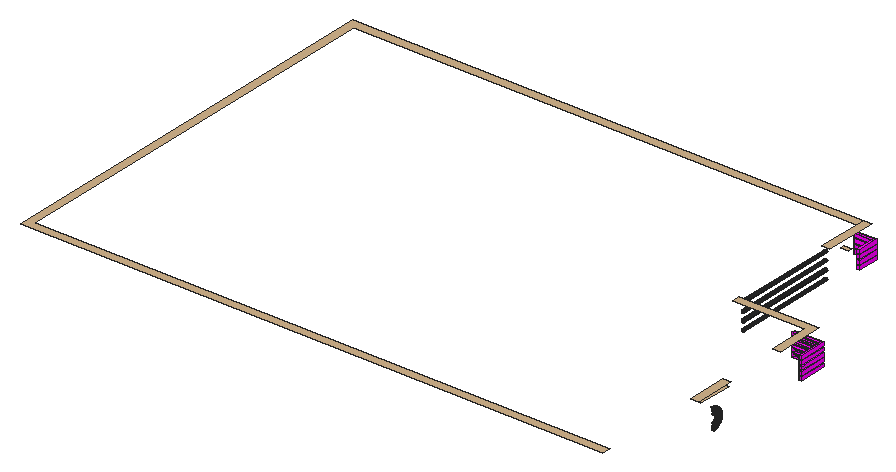
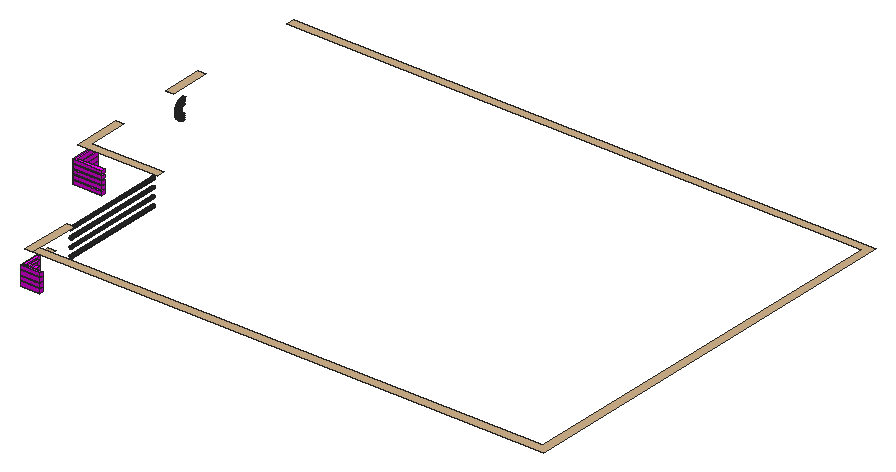
# SketchUp Ruby script. Lengths in inches.
U = 1.inch
M = Sketchup.active_model
def pt(a) = Geom::Point3d.new(a.map { |v| v * U })
def face(e, loops, mat)
  f = e.add_face(loops[0].map { |a| pt(a) })
  loops[1..].each { |l| e.add_face(l.map { |a| pt(a) }).erase! }
  f.material = f.back_material = mat if mat
  f
end
# faces: each face lists its corners as indices into pts; further lists are holes
def faces(e, pts, list, mat = nil) = list.each { |f| face(e, (f[0].is_a?(Array) ? f : [f]).map { |l| l.map { |i| pts[i] } }, mat) }
# xy, xz, yz: faces in a plane at the given z, y or x. An outline is a flat list of corners, or four numbers for a rectangle; further outlines are holes
def ring(l) = l.size == 4 ? [[l[0], l[1]], [l[2], l[1]], [l[2], l[3]], [l[0], l[3]]] : l.each_slice(2).to_a
def flat(e, list, mat, &to3) = list.each { |f| face(e, (f[0].is_a?(Array) ? f : [f]).map { |l| ring(l).map { |u, v| to3.(u, v) } }, mat) }
def xy(e, z, list, mat = nil) = flat(e, list, mat) { |x, y| [x, y, z] }
def xz(e, y, list, mat = nil) = flat(e, list, mat) { |x, z| [x, y, z] }
def yz(e, x, list, mat = nil) = flat(e, list, mat) { |y, z| [x, y, z] }
def lines(e, pts, list) = list.each { |a, b| e.add_line(pt(pts[a]), pt(pts[b])) }
# prism: a flat outline (further loops are holes) pulled along v
def prism(e, loops, v, mat = nil)
  f = face(e, loops, mat); d = Geom::Vector3d.new(v.map { |x| x * U })
  f.pushpull(f.normal.samedirection?(d) ? d.length : -d.length)
end
def box(e, o, s, mat = nil) = prism(e, [[o, [o[0] + s[0], o[1], o[2]], [o[0] + s[0], o[1] + s[1], o[2]], [o[0], o[1] + s[1], o[2]]]], [0, 0, s[2]], mat)
def at(x, y, z, deg = 0) = Geom::Transformation.translation(pt([x, y, z])) * Geom::Transformation.rotation(ORIGIN, Z_AXIS, deg.degrees)
def axes(o, x, y, z) = Geom::Transformation.new([*x, 0, *y, 0, *z, 0, *pt(o).to_a, 1])
def part(name) = M.definitions.add(name)
# library, detail: a bought-in or finely detailed component or shape, given as its bounding box
def library(name, o, s) = part(name).tap { |d| box(d.entities, o, s) }
def detail(e, o, s) = box(e.add_group.entities, o, s)
def put(e, d, t, mat = nil) = e.add_instance(d, t).tap { |i| i.material = mat if mat }
def group(e, t, mat = nil) = e.add_group.tap { |g| g.transformation = t; g.material = mat if mat }.entities
root = M.entities
M.materials.add("[0035_Tan]").color = [210, 180, 140]
M.materials.add("[0127_Magenta]").color = [255, 0, 255]
M.materials.add("[0136_Charcoal]").color = [35, 35, 35]
c1 = part("Component\#10")
xy(c1.entities,0,[[20,0,20,19,0,19,0,21,22,21,22,0]])
xy(c1.entities,2.5625,[[20,0,22,0,22,21,0,21,0,19,20,19]])
xz(c1.entities,0,[[20,0,22,2.5625]])
xz(c1.entities,21,[[0,0,22,2.5625]])
yz(c1.entities,0,[[19,0,21,2.5625]])
yz(c1.entities,20,[[0,0,19,2.5625]])
yz(c1.entities,22,[[0,0,21,2.5625]])
c2 = part("Group\#24")
prism(c2.entities,[[[2.25,1.125,0],[2.21,0.83,0],[2.1,0.5625,0],[1.92,0.33,0],[1.6875,0.15,0],[1.42,0.04,0],[1.125,0,0],[0.83,0.04,0],[0.5625,0.15,0],[0.33,0.33,0],[0.15,0.5625,0],[0.04,0.83,0],[0,1.125,0],[0.04,1.42,0],[0.15,1.6875,0],[0.33,1.92,0],[0.5625,2.1,0],[0.83,2.21,0],[1.125,2.25,0],[1.42,2.21,0],[1.6875,2.1,0],[1.92,1.92,0],[2.1,1.6875,0],[2.21,1.42,0]]],[0,0,77.9])
c3 = part("Component\#2")
xy(c3.entities,-13,[[13.51,0,15.51,2.94]],"[0127_Magenta]")
xy(c3.entities,2,[[0,0,15.51,2.94]],"[0127_Magenta]")
xz(c3.entities,0,[[13.51,-13,15.51,0],[0,0,15.51,2]],"[0127_Magenta]")
xz(c3.entities,2.94,[[13.51,-13,15.51,2],[0,0,13.51,2]],"[0127_Magenta]")
yz(c3.entities,0,[[0,0,2.94,2]],"[0127_Magenta]")
yz(c3.entities,13.51,[[0,-13,2.94,2]],"[0127_Magenta]")
yz(c3.entities,15.51,[[0,-13,2.94,2]],"[0127_Magenta]")
xy(root,161.91,[[442,98.56,443.75,98.95]],"[0035_Tan]")
xy(root,163.37,[[442,98.52,443.75,99]],"[0127_Magenta]")
xy(root,165.21,[[384,292.3,390,295.12]],"[0035_Tan]")
xy(root,172,[[442,86.55,444,112.55]],"[0035_Tan]")
xy(root,174,[[0,2,438,2,438,8,6,8,6,308,384,308,384,314,0,314],[438,84.55,444,114.55],[438,161.1,444,161.1,444,197.1,384,197.1,384,191.1,438,191.1],[384,275,390,314]],"[0035_Tan]")
xz(root,101.97,[[442,155.57,443.5,155.77]],"[0035_Tan]")
xz(root,103.75,[[442,155.51,443.5,155.82]],"[0127_Magenta]")
xz(root,104.99,[[442,155.47,443.75,155.86]],"[0035_Tan]")
xz(root,106.44,[[442,155.42,443.75,155.91]],"[0127_Magenta]")
p = [[442,98.98,147.98],[442,99.47,148.01],[443.75,99.47,148.01],[443.75,98.98,147.98],[442,99.95,148.07],[443.75,99.95,148.07],
  [442,100.42,148.16],[443.75,100.42,148.16],[442,100.89,148.28],[443.75,100.89,148.28],[442,101.35,148.43],[443.75,101.35,148.43],
  [442,101.8,148.61],[443.75,101.8,148.61],[442,102.24,148.8125],[443.75,102.24,148.8125],[442,102.66,149.04],[443.75,102.66,149.04],
  [442,103.07,149.3],[443.75,103.07,149.3],[442,103.46,149.59],[443.75,103.46,149.59],[442,99.33,149.46],[442,98.9375,149.43],
  [443.75,98.9375,149.43],[443.75,99.33,149.46],[442,99.72,149.51],[443.75,99.72,149.51],[442,100.1,149.58],[443.75,100.1,149.58],
  [442,100.48,149.68],[443.75,100.48,149.68],[442,103.83,149.89],[443.75,103.83,149.89],[442,100.86,149.8],[443.75,100.86,149.8],
  [442,101.22,149.94],[443.75,101.22,149.94],[442,101.58,150.11],[443.75,101.58,150.11],[442,104.1875,150.22],[443.75,104.1875,150.22],
  [442,101.92,150.3],[443.75,101.92,150.3],[442,104.52,150.58],[443.75,104.52,150.58],[442,102.25,150.51],[443.75,102.25,150.51],
  [442,102.57,150.74],[443.75,102.57,150.74],[442,104.83,150.95],[443.75,104.83,150.95],[442,98.9,150.68],[442,99.21,150.69],
  [443.5,99.21,150.69],[443.5,98.9,150.68],[442,99.53,150.73],[443.5,99.53,150.73],[442,99.84,150.79],[443.5,99.84,150.79],
  [442,102.87,150.99],[443.75,102.87,150.99],[442,100.14,150.87],[443.5,100.14,150.87],[442,100.4375,150.97],[443.5,100.4375,150.97],
  [442,105.11,151.34],[443.75,105.11,151.34],[442,100.73,151.08],[443.5,100.73,151.08],[442,103.16,151.26],[443.75,103.16,151.26],
  [442,101.01,151.22],[443.5,101.01,151.22],[442,101.29,151.37],[443.5,101.29,151.37],[442,103.43,151.54],[443.75,103.43,151.54],
  [442,105.37,151.75],[443.75,105.37,151.75],[442,101.56,151.53],[443.5,101.56,151.53],[442,101.81,151.72],[443.5,101.81,151.72],
  [442,103.68,151.84],[443.75,103.68,151.84],[442,102.05,151.92],[443.5,102.05,151.92],[442,105.6,152.17],[443.75,105.6,152.17],
  [442,103.91,152.16],[443.75,103.91,152.16],[442,102.28,152.13],[443.5,102.28,152.13],[442,102.5,152.36],[443.5,102.5,152.36],
  [442,104.12,152.49],[443.75,104.12,152.49],[442,105.81,152.61],[443.75,105.81,152.61],[442,99.05,152.46],[442,98.85,152.45],
  [443.5,98.85,152.45],[443.5,99.05,152.46],[442,102.7,152.6],[443.5,102.7,152.6],[442,99.25,152.49],[443.5,99.25,152.49],
  [442,99.45,152.52],[443.5,99.45,152.52],[442,99.65,152.57],[443.5,99.65,152.57],[442,104.31,152.83],[443.75,104.31,152.83],
  [442,99.84,152.64],[443.5,99.84,152.64],[442,100.03,152.71],[443.5,100.03,152.71],[442,102.88,152.86],[443.5,102.88,152.86],
  [442,105.99,153.06],[443.75,105.99,153.06],[442,100.21,152.8],[443.5,100.21,152.8],[442,100.39,152.9],[443.5,100.39,152.9],
  [442,104.47,153.1875],[443.75,104.47,153.1875],[442,100.56,153],[443.5,100.56,153],[442,103.05,153.12],[443.5,103.05,153.12],
  [442,100.72,153.12],[443.5,100.72,153.12],[442,100.88,153.25],[443.5,100.88,153.25],[442,103.2,153.4],[443.5,103.2,153.4],
  [442,106.14,153.52],[443.75,106.14,153.52],[442,104.62,153.55],[443.75,104.62,153.55],[442,101.03,153.39],[443.5,101.03,153.39],
  [442,101.17,153.54],[443.5,101.17,153.54],[442,103.34,153.68],[443.5,103.34,153.68],[442,101.3,153.69],[443.5,101.3,153.69],
  [442,106.26,153.99],[443.75,106.26,153.99],[442,104.74,153.93],[443.75,104.74,153.93],[442,101.41,153.86],[443.5,101.41,153.86],
  [442,103.45,153.97],[443.5,103.45,153.97],[442,101.52,154.03],[443.5,101.52,154.03],[442,104.84,154.3],[443.75,104.84,154.3],
  [442,101.62,154.21],[443.5,101.62,154.21],[442,103.55,154.27],[443.5,103.55,154.27],[442,106.35,154.46],[443.75,106.35,154.46],
  [442,101.71,154.39],[443.5,101.71,154.39],[442,103.63,154.58],[443.5,103.63,154.58],[442,104.91,154.69],[443.75,104.91,154.69],
  [442,101.78,154.58],[443.5,101.78,154.58],[442,106.41,154.94],[443.75,106.41,154.94],[442,101.85,154.77],[443.5,101.85,154.77],
  [442,103.6875,154.89],[443.5,103.6875,154.89],[442,104.96,155.08],[443.75,104.96,155.08],[442,101.9,154.97],[443.5,101.9,154.97],
  [442,103.73,155.2],[443.5,103.73,155.2],[442,106.44,155.42],[443.75,106.44,155.42],[442,101.93,155.16],[443.5,101.93,155.16],
  [442,104.99,155.47],[443.75,104.99,155.47],[442,101.96,155.37],[443.5,101.96,155.37],[442,103.75,155.51],[443.5,103.75,155.51],
  [442,101.97,155.57],[443.5,101.97,155.57],[442,101.96,155.97],[442,101.97,155.77],[443.5,101.97,155.77],[443.5,101.96,155.97],
  [442,103.75,155.82],[442,103.73,156.14],[443.5,103.73,156.14],[443.5,103.75,155.82],[442,104.96,156.25],[442,104.99,155.86],
  [443.75,104.99,155.86],[443.75,104.96,156.25],[442,106.44,155.91],[442,106.41,156.39],[443.75,106.41,156.39],[443.75,106.44,155.91],
  [442,101.94,156.17],[443.5,101.94,156.17],[442,103.6875,156.45],[443.5,103.6875,156.45],[442,101.9,156.37],[443.5,101.9,156.37],
  [442,104.91,156.64],[443.75,104.91,156.64],[442,101.85,156.57],[443.5,101.85,156.57],[442,103.63,156.76],[443.5,103.63,156.76],
  [442,106.35,156.87],[443.75,106.35,156.87],[442,101.78,156.76],[443.5,101.78,156.76],[442,104.84,157.03],[443.75,104.84,157.03],
  [442,101.71,156.95],[443.5,101.71,156.95],[442,103.55,157.0625],[443.5,103.55,157.0625],[442,106.26,157.34],[443.75,106.26,157.34],
  [442,101.625,157.13],[443.5,101.625,157.13],[442,104.74,157.41],[443.75,104.74,157.41],[442,101.53,157.3125],[443.5,101.53,157.3125],
  [442,103.46,157.36],[443.5,103.46,157.36],[442,101.42,157.48],[443.5,101.42,157.48],[442,106.14,157.8125],[443.75,106.14,157.8125],
  [442,103.34,157.65],[443.5,103.34,157.65],[442,104.625,157.78],[443.75,104.625,157.78],[442,101.3,157.65],[443.5,101.3,157.65],
  [442,101.17,157.8],[443.5,101.17,157.8],[442,103.21,157.9375],[443.5,103.21,157.9375],[442,101.03,157.95],[443.5,101.03,157.95],
  [442,104.48,158.15],[443.75,104.48,158.15],[442,105.99,158.27],[443.75,105.99,158.27],[442,103.06,158.21],[443.5,103.06,158.21],
  [442,100.88,158.09],[443.5,100.88,158.09],[442,100.73,158.22],[443.5,100.73,158.22],[442,104.3125,158.5],[443.75,104.3125,158.5],
  [442,100.57,158.34],[443.5,100.57,158.34],[442,102.89,158.48],[443.5,102.89,158.48],[442,100.39,158.45],[443.5,100.39,158.45],
  [442,105.82,158.72],[443.75,105.82,158.72],[442,100.22,158.54],[443.5,100.22,158.54],[442,100.03,158.63],[443.5,100.03,158.63],
  [442,102.7,158.73],[443.5,102.7,158.73],[442,104.125,158.84],[443.75,104.125,158.84],[442,99.85,158.71],[443.5,99.85,158.71],
  [442,99.65,158.77],[443.5,99.65,158.77],[442,102.5,158.98],[443.5,102.5,158.98],[442,105.61,159.16],[443.75,105.61,159.16],
  [442,99.26,158.86],[442,99.46,158.82],[443.5,99.46,158.82],[443.5,99.26,158.86],[442,103.92,159.18],[443.75,103.92,159.18],
  [442,98.85,158.9],[442,99.06,158.88],[443.5,99.06,158.88],[443.5,98.85,158.9],[442,102.29,159.2],[443.5,102.29,159.2],
  [442,102.06,159.42],[443.5,102.06,159.42],[442,103.69,159.49],[443.75,103.69,159.49],[442,105.38,159.58],[443.75,105.38,159.58],
  [442,101.82,159.62],[443.5,101.82,159.62],[442,103.44,159.79],[443.75,103.44,159.79],[442,101.5625,159.81],[443.5,101.5625,159.81],
  [442,105.12,159.99],[443.75,105.12,159.99],[442,101.3,159.97],[443.5,101.3,159.97],[442,103.17,160.08],[443.75,103.17,160.08],
  [442,101.02,160.125],[443.5,101.02,160.125],[442,104.84,160.38],[443.75,104.84,160.38],[442,100.74,160.26],[443.5,100.74,160.26],
  [442,102.88,160.35],[443.75,102.88,160.35],[442,100.45,160.375],[443.5,100.45,160.375],[442,102.58,160.6],[443.75,102.58,160.6],
  [442,100.15,160.47],[443.5,100.15,160.47],[442,104.53,160.76],[443.75,104.53,160.76],[442,99.85,160.55],[443.5,99.85,160.55],
  [442,99.54,160.61],[442,99.23,160.65],[443.5,99.23,160.65],[443.5,99.54,160.61],[442,102.26,160.83],[443.75,102.26,160.83],
  [442,98.91,160.67],[443.5,98.91,160.67],[442,101.93,161.04],[443.75,101.93,161.04],[442,104.2,161.11],[443.75,104.2,161.11],
  [442,101.59,161.23],[443.75,101.59,161.23],[442,103.85,161.44],[443.75,103.85,161.44],[442,101.23,161.4],[443.75,101.23,161.4],
  [442,100.87,161.54],[443.75,100.87,161.54],[442,103.47,161.75],[443.75,103.47,161.75],[442,100.5,161.66],[443.75,100.5,161.66],
  [442,100.12,161.76],[443.75,100.12,161.76],[442,103.08,162.03],[443.75,103.08,162.03],[442,99.34,161.89],[442,99.73,161.84],
  [443.75,99.73,161.84],[443.75,99.34,161.89],[442,98.95,161.91],[443.75,98.95,161.91],[442,102.67,162.29],[443.75,102.67,162.29],
  [442,102.25,162.53],[443.75,102.25,162.53],[442,101.8125,162.73],[443.75,101.8125,162.73],[442,101.36,162.91],[443.75,101.36,162.91],
  [442,100.9,163.0625],[443.75,100.9,163.0625],[442,100.4375,163.18],[443.75,100.4375,163.18],[442,99.96,163.27],[443.75,99.96,163.27],
  [442,99.48,163.33],[442,99,163.37],[443.75,99,163.37],[443.75,99.48,163.33]]
faces(root,p,[[0,1,2,3],[1,4,5,2],[4,6,7,5],[6,8,9,7],[8,10,11,9],[10,12,13,11],[12,14,15,13],[14,16,17,15],
  [16,18,19,17],[18,20,21,19],[20,32,33,21],[32,40,41,33],[40,44,45,41],[44,50,51,45],[52,53,54,55],[53,56,57,54],
  [56,58,59,57],[58,62,63,59],[62,64,65,63],[50,66,67,51],[64,68,69,65],[68,72,73,69],[72,74,75,73],[66,78,79,67],
  [74,80,81,75],[80,82,83,81],[82,86,87,83],[78,88,89,79],[86,92,93,87],[92,94,95,93],[88,98,99,89],[94,104,105,95],
  [104,118,119,105],[98,120,121,99],[118,130,131,119],[130,136,137,131],[120,138,139,121],[136,146,147,137],[138,150,151,139],[146,156,157,147],
  [156,164,165,157],[150,166,167,151],[164,170,171,165],[166,176,177,167],[170,180,181,171],[180,186,187,181],[176,188,189,177],[186,196,197,187],
  [204,205,206,207],[212,213,214,215],[205,218,219,206],[218,226,227,219],[213,228,229,214],[226,236,237,227],[228,238,239,229],[236,246,247,237],
  [238,250,251,239],[246,252,253,247],[252,260,261,253],[250,266,267,251],[260,268,269,261],[268,278,279,269],[266,282,283,267],[278,288,289,279],
  [288,296,297,289],[282,298,299,283],[296,310,311,297],[310,312,313,311],[298,316,317,299],[312,318,319,313],[318,322,323,319],[316,324,325,317],
  [322,326,327,323],[326,330,331,327],[324,332,333,325],[330,334,335,331],[334,338,339,335],[338,342,343,339],[332,344,345,333],[342,346,347,343],
  [348,349,350,351],[346,348,351,347],[349,354,355,350],[344,358,359,345],[358,362,363,359],[362,368,369,363],[368,374,375,369],[374,382,383,375],
  [382,384,385,383],[384,386,387,385],[386,388,389,387],[388,390,391,389],[390,392,393,391],[392,394,395,393],[396,397,398,399],[394,396,399,395]],"[0127_Magenta]")
faces(root,p,[[22,23,24,25],[26,22,25,27],[28,26,27,29],[30,28,29,31],[34,30,31,35],[36,34,35,37],[38,36,37,39],[42,38,39,43],
  [46,42,43,47],[48,46,47,49],[60,48,49,61],[70,60,61,71],[76,70,71,77],[84,76,77,85],[90,84,85,91],[96,90,91,97],
  [100,101,102,103],[106,100,103,107],[108,106,107,109],[110,108,109,111],[112,96,97,113],[114,110,111,115],[116,114,115,117],[122,116,117,123],
  [124,122,123,125],[126,112,113,127],[128,124,125,129],[132,128,129,133],[134,132,133,135],[140,126,127,141],[142,134,135,143],[144,142,143,145],
  [148,144,145,149],[152,140,141,153],[154,148,149,155],[158,154,155,159],[160,152,153,161],[162,158,159,163],[168,162,163,169],[172,160,161,173],
  [174,168,169,175],[178,174,175,179],[182,172,173,183],[184,178,179,185],[190,184,185,191],[192,182,183,193],[194,190,191,195],[198,194,195,199],
  [200,201,202,203],[208,209,210,211],[216,200,203,217],[220,216,217,221],[222,208,211,223],[224,220,221,225],[230,224,225,231],[232,222,223,233],
  [234,230,231,235],[240,234,235,241],[242,232,233,243],[244,240,241,245],[248,244,245,249],[254,242,243,255],[256,248,249,257],[258,256,257,259],
  [262,258,259,263],[264,254,255,265],[270,262,263,271],[272,270,271,273],[274,264,265,275],[276,272,273,277],[280,276,277,281],[284,280,281,285],
  [286,284,285,287],[290,274,275,291],[292,286,287,293],[294,292,293,295],[300,301,302,303],[301,294,295,302],[304,290,291,305],[306,307,308,309],
  [307,300,303,308],[314,304,305,315],[320,314,315,321],[328,320,321,329],[336,328,329,337],[340,336,337,341],[352,340,341,353],[356,352,353,357],
  [360,356,357,361],[364,360,361,365],[366,364,365,367],[370,366,367,371],[372,370,371,373],[376,377,378,379],[377,372,373,378],[380,376,379,381]],"[0035_Tan]")
put(root,c1,at(424,178.1,147.625),"[0127_Magenta]")
put(root,c1,at(424,178.1,151.1875),"[0127_Magenta]")
put(root,c1,at(424,178.1,154.75),"[0127_Magenta]")
put(root,c1,at(424,178.1,158.3125),"[0127_Magenta]")
put(root,c1,at(424,178.1,161.875),"[0127_Magenta]")
put(root,c2,axes([385.75,275,151.51],[1,0,0],[0,0,1],[0,-1,0]),"[0136_Charcoal]")
put(root,c2,axes([385.75,275,157.84],[1,0,0],[0,0,1],[0,-1,0]),"[0136_Charcoal]")
put(root,c2,axes([385.75,275,164.17],[1,0,0],[0,0,1],[0,-1,0]),"[0136_Charcoal]")
put(root,c2,axes([385.75,275,170.5],[1,0,0],[0,0,1],[0,-1,0]),"[0136_Charcoal]")
put(root,c3,axes([390,300.49,149.41],[0,1,0],[0,0,1],[1,0,0]))
put(root,c3,axes([390,300.49,153.1],[0,1,0],[0,0,1],[1,0,0]))
put(root,c3,axes([390,300.49,156.79],[0,1,0],[0,0,1],[1,0,0]))
put(root,c3,axes([390,300.49,160.47],[0,1,0],[0,0,1],[1,0,0]))
